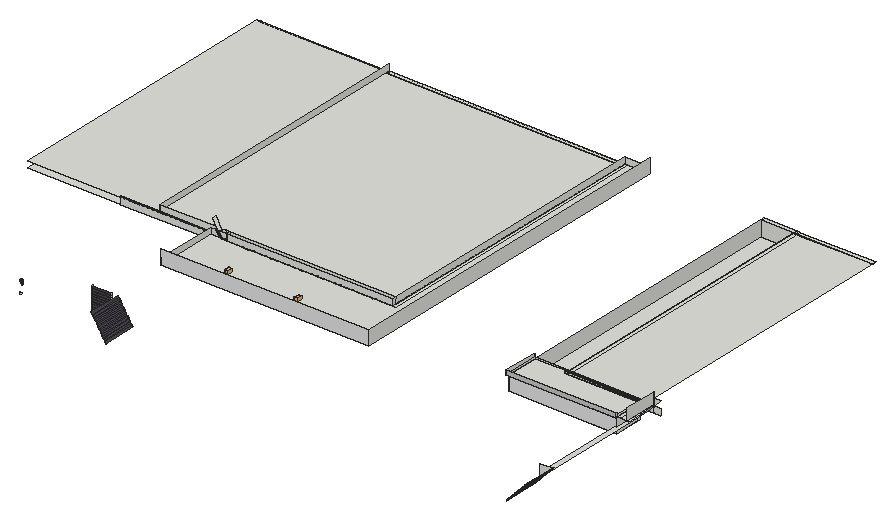
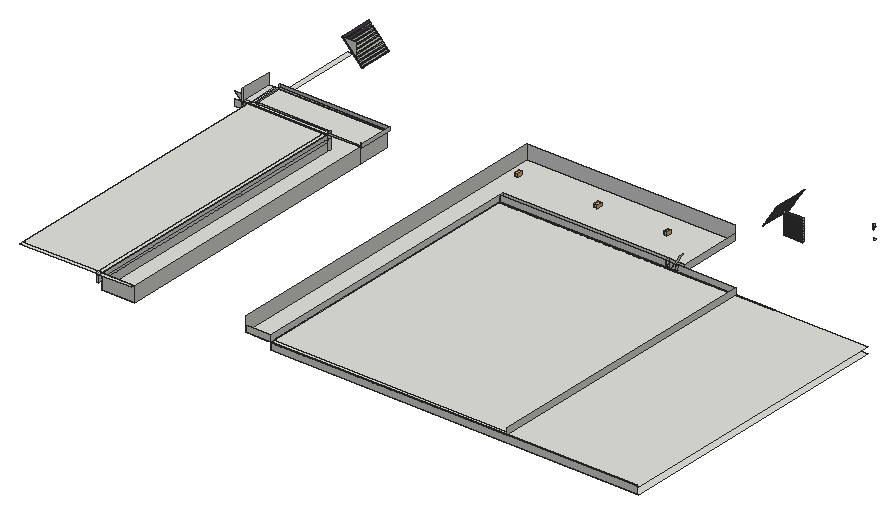
# SketchUp Ruby script. Lengths in inches.
U = 1.inch
M = Sketchup.active_model
def pt(a) = Geom::Point3d.new(a.map { |v| v * U })
def face(e, loops, mat)
  f = e.add_face(loops[0].map { |a| pt(a) })
  loops[1..].each { |l| e.add_face(l.map { |a| pt(a) }).erase! }
  f.material = f.back_material = mat if mat
  f
end
# faces: each face lists its corners as indices into pts; further lists are holes
def faces(e, pts, list, mat = nil) = list.each { |f| face(e, (f[0].is_a?(Array) ? f : [f]).map { |l| l.map { |i| pts[i] } }, mat) }
# xy, xz, yz: faces in a plane at the given z, y or x. An outline is a flat list of corners, or four numbers for a rectangle; further outlines are holes
def ring(l) = l.size == 4 ? [[l[0], l[1]], [l[2], l[1]], [l[2], l[3]], [l[0], l[3]]] : l.each_slice(2).to_a
def flat(e, list, mat, &to3) = list.each { |f| face(e, (f[0].is_a?(Array) ? f : [f]).map { |l| ring(l).map { |u, v| to3.(u, v) } }, mat) }
def xy(e, z, list, mat = nil) = flat(e, list, mat) { |x, y| [x, y, z] }
def xz(e, y, list, mat = nil) = flat(e, list, mat) { |x, z| [x, y, z] }
def yz(e, x, list, mat = nil) = flat(e, list, mat) { |y, z| [x, y, z] }
def lines(e, pts, list) = list.each { |a, b| e.add_line(pt(pts[a]), pt(pts[b])) }
# prism: a flat outline (further loops are holes) pulled along v
def prism(e, loops, v, mat = nil)
  f = face(e, loops, mat); d = Geom::Vector3d.new(v.map { |x| x * U })
  f.pushpull(f.normal.samedirection?(d) ? d.length : -d.length)
end
def box(e, o, s, mat = nil) = prism(e, [[o, [o[0] + s[0], o[1], o[2]], [o[0] + s[0], o[1] + s[1], o[2]], [o[0], o[1] + s[1], o[2]]]], [0, 0, s[2]], mat)
def at(x, y, z, deg = 0) = Geom::Transformation.translation(pt([x, y, z])) * Geom::Transformation.rotation(ORIGIN, Z_AXIS, deg.degrees)
def axes(o, x, y, z) = Geom::Transformation.new([*x, 0, *y, 0, *z, 0, *pt(o).to_a, 1])
def part(name) = M.definitions.add(name)
# library, detail: a bought-in or finely detailed component or shape, given as its bounding box
def library(name, o, s) = part(name).tap { |d| box(d.entities, o, s) }
def detail(e, o, s) = box(e.add_group.entities, o, s)
def put(e, d, t, mat = nil) = e.add_instance(d, t).tap { |i| i.material = mat if mat }
def group(e, t, mat = nil) = e.add_group.tap { |g| g.transformation = t; g.material = mat if mat }.entities
root = M.entities
M.materials.add("[Color M01]").color = [226, 226, 226]
M.materials.add("[Color M02]").color = [198, 198, 198]
M.materials.add("[Color M06]").color = [79, 71, 84]
c1 = library("Group\#13",[0,0,0],[3.54,3.54,3.9375])
xy(root,306.39,[[578.05,523.75,609.02,526.125]])
xy(root,307.2,[[578.05,523.75,609.02,526.125]])
xy(root,310.33,[[578.05,523.75,609.02,526.125]])
xy(root,311.14,[[578.05,523.75,609.02,526.125]])
xy(root,314.27,[[578.05,523.75,609.02,526.125]])
xy(root,315.08,[[578.05,524.25,609.02,526.125]])
xy(root,315.25,[[1139.11,678.64,1139.11,1195.68,1192.67,1195.68,1192.67,726.125,1316.04,726.125,1316.04,678.64]])
xy(root,318.2,[[578.05,524.25,609.02,526.125]])
xy(root,319.01,[[578.05,524.25,609.02,526.125]])
xy(root,322.14,[[578.05,524.25,609.02,526.125]])
xy(root,322.89,[[578.05,524.25,609.02,526.125]])
xy(root,326.02,[[578.05,524.25,609.02,526.125]])
xy(root,326.08,[[1314.46,528.48,1322.96,719.2],[1314.46,719.2,1322.96,719.59]])
xy(root,326.76,[[578.05,524.25,609.02,526.125]])
xy(root,328,[[306.21,732.2,910.57,1201.875]])
xy(root,329.89,[[578.05,524.25,609.02,526.125]])
xy(root,330.64,[[578.05,524.25,609.02,526.125]])
xy(root,333.125,[[1192.67,726.125,1196.48,732.2],[1192.67,732.2,1196.48,734.4375],[1192.67,734.4375,1196.48,1195.68]])
xy(root,333.71,[[497.26,480.14,499.58,480.77]])
xy(root,333.77,[[578.05,524.25,609.02,526.125]])
xy(root,334.51,[[578.05,524.25,609.02,526.125]])
xy(root,336.02,[[497.26,480.14,499.58,480.77]])
xy(root,336.52,[[497.26,480.14,499.58,480.77]])
xy(root,337.64,[[578.05,524.25,609.02,526.125]])
xy(root,338.39,[[578.05,524.25,609.02,526.125]])
xy(root,338.84,[[494.35,480.14,496.66,480.77],[497.26,480.14,499.58,480.77]])
xy(root,338.875,[[306.21,732.2,910.57,1201.875]])
xy(root,339.34,[[494.35,480.14,496.66,480.77],[497.26,480.14,499.58,480.77]])
xy(root,340.125,[[611.36,623.84,611.36,726.125,663.69,726.125,663.69,724.8125,669.77,724.8125,669.77,726.125,673.19,726.125,673.19,724.8125,679.27,724.8125,679.27,726.125,682.69,726.125,682.69,724.8125,688.77,724.8125,688.77,726.125,692.19,726.125,692.19,724.8125,698.27,724.8125,698.27,726.125,701.69,726.125,701.69,724.8125,707.77,724.8125,707.77,726.125,711.19,726.125,711.19,724.8125,717.27,724.8125,717.27,726.125,720.69,726.125,720.69,724.8125,726.77,724.8125,726.77,726.125,730.19,726.125,730.19,724.8125,736.27,724.8125,736.27,726.125,739.69,726.125,739.69,724.8125,745.77,724.8125,745.77,726.125,749.19,726.125,749.19,724.8125,755.27,724.8125,755.27,726.125,758.69,726.125,758.69,724.8125,764.77,724.8125,764.77,726.125,768.19,726.125,768.19,724.8125,774.27,724.8125,774.27,726.125,777.69,726.125,777.69,724.8125,783.77,724.8125,783.77,726.125,787.19,726.125,787.19,724.8125,793.27,724.8125,793.27,726.125,796.69,726.125,796.69,724.8125,802.77,724.8125,802.77,726.125,806.19,726.125,806.19,724.8125,812.27,724.8125,812.27,726.125,815.69,726.125,815.69,724.8125,821.77,724.8125,821.77,726.125,825.19,726.125,825.19,724.8125,831.27,724.8125,831.27,726.125,834.69,726.125,834.69,724.8125,840.77,724.8125,840.77,726.125,844.19,726.125,844.19,724.8125,850.27,724.8125,850.27,726.125,853.69,726.125,853.69,724.8125,859.77,724.8125,859.77,726.125,863.19,726.125,863.19,724.8125,869.27,724.8125,869.27,726.125,872.69,726.125,872.69,724.8125,878.77,724.8125,878.77,726.125,882.19,726.125,882.19,724.8125,888.27,724.8125,888.27,726.125,891.69,726.125,891.69,724.8125,897.77,724.8125,897.77,726.125,901.19,726.125,901.19,724.8125,907.27,724.8125,907.27,726.125,910.69,726.125,910.69,724.8125,916.77,724.8125,916.77,1201.875,952.01,1201.875,952.01,623.84],[1136.54,676.08,1139.11,678.64],[1139.11,676.08,1316.04,678.64],[1136.54,678.64,1139.11,732.2],[1139.11,678.64,1139.11,732.2,1192.67,732.2,1192.67,726.125,1316.04,726.125,1316.04,678.64],
  [1316.04,678.64,1322.24,726.125],[1322.24,678.64,1322.96,726.125],[1322.96,678.64,1333.34,726.125],[1333.34,678.64,1336.18,726.125],[663.69,724.8125,669.77,726.125],
  [673.19,724.8125,679.27,726.125],[682.69,724.8125,688.77,726.125],[692.19,724.8125,698.27,726.125],[701.69,724.8125,707.77,726.125],[711.19,724.8125,717.27,726.125],
  [720.69,724.8125,726.77,726.125],[730.19,724.8125,736.27,726.125],[739.69,724.8125,745.77,726.125],[749.19,724.8125,755.27,726.125],[758.69,724.8125,764.77,726.125],
  [768.19,724.8125,774.27,726.125],[777.69,724.8125,783.77,726.125],[787.19,724.8125,793.27,726.125],[796.69,724.8125,802.77,726.125],[806.19,724.8125,812.27,726.125],
  [815.69,724.8125,821.77,726.125],[825.19,724.8125,831.27,726.125],[834.69,724.8125,840.77,726.125],[844.19,724.8125,850.27,726.125],[853.69,724.8125,859.77,726.125],
  [863.19,724.8125,869.27,726.125],[872.69,724.8125,878.77,726.125],[882.19,724.8125,888.27,726.125],[891.69,724.8125,897.77,726.125],[901.19,724.8125,907.27,726.125],
  [910.69,724.8125,916.77,1201.875],[637.42,726.125,910.57,732.2],[910.57,726.125,910.69,732.2],[1192.67,726.125,1198.75,732.2],[1198.75,726.125,1322.24,732.2],
  [1322.96,726.125,1333.34,732.2],[1333.34,726.125,1336.18,732.2],[522.625,732.2,637.42,734.4375],[637.42,732.2,910.57,734.4375],[910.57,732.2,910.69,734.4375],
  [1192.67,732.2,1198.75,734.4375],[1198.75,732.2,1322.24,732.2,1322.24,732.32,1198.87,732.32,1198.87,734.4375,1198.75,734.4375],[1322.24,732.2,1322.96,734.4375],[1198.87,732.32,1322.24,734.4375],[522.625,734.4375,910.57,1195.68],
  [910.57,734.4375,910.69,1195.8],[1192.67,734.4375,1198.75,1195.68],[1198.75,734.4375,1198.87,1195.68],[1198.87,734.4375,1322.24,1195.68],[1322.24,734.4375,1322.96,1195.68],
  [522.625,1195.68,910.57,1195.8],[1139.11,1195.68,1192.67,1195.8],[1192.67,1195.68,1196.48,1195.8],[1192.67,1195.68,1196.48,1195.8],[1196.48,1195.68,1198.75,1195.8],
  [1198.75,1195.68,1322.24,1195.8],[1322.24,1195.68,1322.96,1195.8],[522.625,1195.8,910.57,1201.875],[910.57,1195.8,910.69,1201.875],[1139.11,1195.8,1192.67,1201.875],
  [1192.67,1195.8,1196.48,1201.875],[1196.48,1195.8,1198.75,1201.875],[1198.75,1195.8,1322.24,1201.875],[1322.24,1195.8,1322.96,1201.875]])
xz(root,480.7,[[494.35,319.65,496.66,321.96]])
xz(root,521.5625,[[646.07,305.32,646.4375,305.56,644.74,308.2,644.375,307.97],[1305.53,306.65,1305.08,307.08,1307.5,309.65,1307.95,309.22],[1305.08,307.08,1304.85,307.29,1307.27,309.87,1307.5,309.65],[643.84,308.8,644.21,309.03,642.52,311.68,642.15,311.44],[1308.83,310.16,1308.375,310.59,1310.8,313.16,1311.25,312.73],
  [641.62,312.27,641.98,312.51,640.29,315.15,639.92,314.91],[1312.13,313.66,1311.68,314.09,1314.1,316.66,1314.55,316.23],[639.39,315.74,639.76,315.98,638.0625,318.62,637.7,318.38],[1315.43,317.17,1314.97,317.59,1316.04,318.73,1316.04,317.82],[1316.04,317.82,1316.5,318.3,1316.04,318.73],
  [1316.5,318.3,1317.85,319.74,1317.39,320.17,1316.04,318.73],[1316.04,318.73,1317.39,320.17,1318.27,321.1,1320.69,323.67,1321.57,324.6,1322.96,326.08,1323.99,327.17,1324.87,328.11,1327.29,330.68,1328.17,331.61,1330.59,334.18,1331.47,335.11,1333.89,337.6875,1334.76,338.62,1336.18,340.125,1316.04,340.125],[637.16,319.21,637.53,319.45,635.84,322.09,635.47,321.86],[1318.73,320.67,1321.15,323.24,1320.69,323.67,1318.27,321.1],[634.9375,322.6875,635.31,322.92,633.61,325.57,633.24,325.33],
  [1322.03,324.17,1321.57,324.6,1322.96,326.08,1322.96,325.17],[1322.96,325.17,1322.96,326.08,1323.42,325.65],[1323.42,325.65,1324.45,326.75,1323.99,327.17,1322.96,326.08],[632.71,326.16,633.08,326.4,631.39,329.04,631.02,328.8],[1325.32,327.68,1327.75,330.25,1327.29,330.68,1324.87,328.11],
  [630.48,329.63,630.85,329.87,629.16,332.51,628.79,332.28],[1328.62,331.18,1331.04,333.75,1330.59,334.18,1328.17,331.61],[628.26,333.11,628.625,333.34,626.93,335.98,626.5625,335.75],[1331.92,334.6875,1334.34,337.26,1333.89,337.6875,1331.47,335.11],[626.03,336.58,626.4,336.8125,624.71,339.46,624.34,339.22],
  [1335.22,338.19,1336.64,339.7,1336.18,340.125,1334.76,338.62],[1336.64,339.7,1337.04,340.125,1336.18,340.125],[623.81,340.05,624.17,340.29,622.48,342.93,622.11,342.69],[1336.18,340.125,1337.04,340.125,1337.64,340.76,1337.1875,341.19]])
xz(root,523.75,[[578.05,307.2,609.02,310.33],[578.05,311.14,609.02,314.27]],"[Color M06]")
xz(root,524.25,[[578.05,315.08,609.02,318.2],[578.05,319.01,609.02,322.14],[578.05,322.89,609.02,326.02],[578.05,326.76,609.02,329.89],[578.05,330.64,609.02,333.77],
  [578.05,334.51,609.02,337.64],[578.05,338.39,609.02,341.52]],"[Color M06]")
xz(root,526.125,[[578.05,306.39,609.02,307.2],[578.05,310.33,609.02,311.14],[578.05,314.27,609.02,315.08],[578.05,318.2,609.02,319.01],[578.05,322.14,609.02,322.89],
  [578.05,326.02,609.02,326.76],[578.05,329.89,609.02,330.64],[578.05,333.77,609.02,334.51],[578.05,337.64,609.02,338.39]])
xz(root,623.84,[[611.36,340.125,952.01,363.75]],"[Color M01]")
xz(root,676.08,[[1136.54,340.125,1316.04,346.3125]],"[Color M02]")
xz(root,678.64,[[1139.11,340.125,1316.04,342.6875]])
xz(root,678.64,[[1139.11,315.25,1316.04,340.125]],"[Color M01]")
xz(root,726.125,[[1192.67,315.25,1196.48,333.125],[1196.48,315.25,1198.75,315.25,1198.75,340.125,1192.67,340.125,1192.67,333.125,1196.48,333.125],[1198.75,315.25,1310.86,340.125],[1310.86,315.25,1316.04,340.125],[611.36,340.125,611.36,350.1875,617.83,350.1875,624.28,340.125],
  [624.28,340.125,629.99,340.125,623.54,350.1875,617.83,350.1875],[629.99,340.125,623.54,350.1875,637.42,350.1875,637.42,340.125,635.26,343.5],[629.99,340.125,635.26,343.5,637.42,340.125],[637.42,340.125,910.57,350.1875],[1192.67,340.125,1198.75,342.6875],
  [1198.75,340.125,1310.86,342.6875],[1310.86,340.125,1316.04,342.6875]])
xz(root,732.2,[[1322.96,326.08,1322.96,328,1324.77,328],[459.19,328,617.83,338.875],[617.83,328,623.54,338.875],[623.54,328,630.97,328,630.97,329.69,625.08,338.875,623.54,338.875],[630.97,328,632.05,328,630.97,329.69],
  [632.05,328,637.42,328,637.42,338.875,630.97,338.875,630.97,329.69],[637.42,328,910.57,338.875],[1192.67,328,1198.75,338.875],[1198.75,328,1322.96,338.875],[1322.96,328,1322.96,338.875,1333.34,338.875,1333.34,337.11,1324.77,328],
  [1324.77,328,1333.34,328,1333.34,337.11],[1333.34,328,1345.65,328,1345.65,338.875,1335.01,338.875,1333.34,337.11],[630.97,329.69,630.97,338.875,625.08,338.875],[1333.34,337.11,1333.34,338.875,1335.01,338.875],[459.19,338.875,617.83,340.125],
  [617.83,338.875,623.54,340.125],[623.54,338.875,625.08,338.875,624.28,340.125,623.54,340.125],[625.08,338.875,630.97,338.875,630.97,340.125,624.28,340.125],[630.97,338.875,637.42,340.125],[637.42,338.875,910.57,340.125],
  [1192.67,338.875,1198.75,340.125],[1198.75,338.875,1322.96,340.125],[1322.96,338.875,1333.34,340.125],[1333.34,338.875,1333.34,340.125,1336.18,340.125,1335.01,338.875],[522.625,340.125,617.83,350.1875],
  [617.83,340.125,623.54,340.125,623.54,341.27,617.83,350.1875],[623.54,340.125,624.28,340.125,623.54,341.27],[624.28,340.125,629.99,340.125,623.54,350.1875,623.54,341.27],[629.99,340.125,630.97,340.75,630.97,350.1875,623.54,350.1875],[629.99,340.125,630.97,340.125,630.97,340.75],
  [630.97,340.125,637.42,340.125,637.42,350.1875,630.97,350.1875,635.26,343.5,630.97,340.75],[637.42,340.125,910.57,350.1875],[1136.54,340.125,1139.11,346.3125],[1139.11,340.125,1192.67,342.6875],[1333.34,340.125,1333.34,350.1875,1345.65,350.1875,1336.18,340.125]])
xz(root,1195.68,[[1139.11,315.25,1192.67,340.125],[1192.67,333.125,1196.48,340.125]])
xz(root,1201.875,[[310.02,328,910.57,338.875],[1192.67,328,1196.48,338.875],[310.02,338.875,910.57,340.125],[1192.67,338.875,1196.48,340.125],[910.57,340.125,952.01,350.1875]])
yz(root,496.66,[[480.14,336.52,480.77,338.84],[480.14,339.34,480.77,341.65]])
yz(root,497.26,[[480.14,336.52,480.77,338.84],[480.14,339.34,480.77,341.65]])
yz(root,499.58,[[480.14,336.52,480.77,338.84],[480.14,339.34,480.77,341.65]])
yz(root,522.625,[[732.2,340.125,1201.875,350.1875]])
yz(root,578.05,[[523.75,307.2,526.125,310.33],[523.75,311.14,526.125,314.27],[524.25,315.08,526.125,318.2],[524.25,319.01,526.125,322.14],[524.25,322.89,526.125,326.02],
  [524.25,326.76,526.125,329.89],[524.25,330.64,526.125,333.77],[524.25,334.51,526.125,337.64],[524.25,338.39,526.125,341.52]])
yz(root,609.02,[[523.75,307.2,526.125,310.33],[523.75,311.14,526.125,314.27],[524.25,315.08,526.125,318.2],[524.25,319.01,526.125,322.14],[524.25,322.89,526.125,326.02],
  [524.25,326.76,526.125,329.89],[524.25,330.64,526.125,333.77],[524.25,334.51,526.125,337.64],[524.25,338.39,526.125,341.52]])
yz(root,611.36,[[623.84,340.125,726.125,350.1875]])
yz(root,637.42,[[726.125,340.125,732.2,350.1875]])
yz(root,910.57,[[732.2,328,1195.68,338.875],[1195.68,328,1201.875,338.875],[732.2,338.875,1195.68,340.125],[1195.68,338.875,1201.875,340.125],[726.125,340.125,732.2,350.1875],
  [732.2,340.125,1201.875,350.1875]])
yz(root,952.01,[[623.84,340.125,1201.875,363.75]])
yz(root,1136.54,[[676.08,340.125,732.2,346.3125]])
yz(root,1139.11,[[678.64,315.25,732.2,340.125],[732.2,315.25,1195.68,340.125],[678.64,340.125,732.2,342.6875]])
yz(root,1192.67,[[726.125,315.25,732.2,333.125],[732.2,315.25,734.4375,328],[734.4375,315.25,1195.68,328],[732.2,328,734.4375,333.125],[734.4375,328,1195.68,333.125],
  [1195.68,328,1201.875,338.875],[726.125,333.125,732.2,340.125],[732.2,333.125,734.4375,338.875],[734.4375,333.125,1195.68,338.875],[732.2,338.875,734.4375,340.125],
  [734.4375,338.875,1195.68,340.125],[1195.68,338.875,1201.875,340.125],[726.125,340.125,732.2,342.6875]])
yz(root,1316.04,[[678.64,315.25,719.59,340.125],[719.59,315.25,726.125,340.125],[676.08,340.125,678.64,346.3125],[678.64,340.125,719.59,342.6875],[719.59,340.125,726.125,342.6875]])
yz(root,1322.96,[[726.125,326.08,732.2,340.125]])
yz(root,1333.34,[[678.64,340.125,731.75,358.5],[731.75,340.125,732.2,358.5]])
p = [[644.375,521.5625,307.97],[646.07,521.5625,305.32],[646.07,467.1875,305.32],[644.375,467.1875,307.97],[646.4375,521.5625,305.56],[646.4375,467.1875,305.56],
  [1304.2,521.5625,306.15],[1304.2,467.1875,306.15],[1304.66,467.1875,305.72],[1304.66,521.5625,305.72],[1303.97,521.5625,306.36],[1303.97,467.1875,306.36],
  [1305.08,521.5625,307.08],[1305.08,467.1875,307.08],[1305.53,521.5625,306.65],[1305.53,467.1875,306.65],[1307.95,521.5625,309.22],[1307.95,467.1875,309.22],
  [1304.85,467.1875,307.29],[1304.85,521.5625,307.29],[1307.5,521.5625,309.65],[1307.5,467.1875,309.65],[1307.27,521.5625,309.87],[1307.27,467.1875,309.87],
  [644.74,467.1875,308.2],[644.74,521.5625,308.2],[644.21,467.1875,309.03],[644.21,521.5625,309.03],[642.15,521.5625,311.44],[643.84,521.5625,308.8],
  [643.84,467.1875,308.8],[642.15,467.1875,311.44],[1308.375,521.5625,310.59],[1308.375,467.1875,310.59],[1308.83,521.5625,310.16],[1308.83,467.1875,310.16],
  [1311.25,521.5625,312.73],[1311.25,467.1875,312.73],[1310.8,521.5625,313.16],[1310.8,467.1875,313.16],[642.52,467.1875,311.68],[642.52,521.5625,311.68],
  [641.98,467.1875,312.51],[641.98,521.5625,312.51],[639.92,521.5625,314.91],[641.62,521.5625,312.27],[641.62,467.1875,312.27],[639.92,467.1875,314.91],
  [1311.68,521.5625,314.09],[1311.68,467.1875,314.09],[1312.13,521.5625,313.66],[1312.13,467.1875,313.66],[1314.55,521.5625,316.23],[1314.55,467.1875,316.23],
  [1314.1,521.5625,316.66],[1314.1,467.1875,316.66],[640.29,467.1875,315.15],[640.29,521.5625,315.15],[639.76,467.1875,315.98],[639.76,521.5625,315.98],
  [637.7,521.5625,318.38],[639.39,521.5625,315.74],[639.39,467.1875,315.74],[637.7,467.1875,318.38],[1314.97,521.5625,317.59],[1314.97,467.1875,317.59],
  [1315.43,521.5625,317.17],[1315.43,467.1875,317.17],[1316.5,521.5625,318.3],[1317.85,521.5625,319.74],[1317.85,467.1875,319.74],[1316.04,521.5625,317.82],
  [1317.39,521.5625,320.17],[1316.04,521.5625,318.73],[1317.39,467.1875,320.17],[638.0625,467.1875,318.62],[638.0625,521.5625,318.62],[637.53,467.1875,319.45],
  [637.53,521.5625,319.45],[635.47,521.5625,321.86],[637.16,521.5625,319.21],[637.16,467.1875,319.21],[635.47,467.1875,321.86],[1318.27,521.5625,321.1],
  [1318.27,467.1875,321.1],[1318.73,521.5625,320.67],[1318.73,467.1875,320.67],[1321.15,521.5625,323.24],[1321.15,467.1875,323.24],[1320.69,521.5625,323.67],
  [1320.69,467.1875,323.67],[635.84,467.1875,322.09],[635.84,521.5625,322.09],[635.31,467.1875,322.92],[635.31,521.5625,322.92],[633.24,521.5625,325.33],
  [634.9375,521.5625,322.6875],[634.9375,467.1875,322.6875],[633.24,467.1875,325.33],[1321.57,521.5625,324.6],[1321.57,467.1875,324.6],[1322.03,521.5625,324.17],
  [1322.03,467.1875,324.17],[1323.42,521.5625,325.65],[1324.45,521.5625,326.75],[1324.45,467.1875,326.75],[1322.96,521.5625,325.17],[1323.99,521.5625,327.17],
  [1322.96,521.5625,326.08],[1323.99,467.1875,327.17],[633.61,467.1875,325.57],[633.61,521.5625,325.57],[633.08,467.1875,326.4],[633.08,521.5625,326.4],
  [1322.96,719.59,326.08],[1322.96,719.2,326.08],[1312.29,719.2,336.13],[1312.29,731.75,336.13],[1322.96,731.75,326.08],[1322.96,726.125,326.08],
  [1336.18,719.59,340.125],[1336.18,726.125,340.125],[1336.18,731.75,340.125],[1336.18,732.2,340.125],[1335.01,732.2,338.875],[1333.34,732.2,337.11],
  [1324.77,732.2,328],[1322.96,732.2,326.08],[631.02,521.5625,328.8],[632.71,521.5625,326.16],[632.71,467.1875,326.16],[631.02,467.1875,328.8],
  [1324.87,521.5625,328.11],[1324.87,467.1875,328.11],[1325.32,521.5625,327.68],[1325.32,467.1875,327.68],[1327.75,521.5625,330.25],[1327.75,467.1875,330.25],
  [1327.29,521.5625,330.68],[1327.29,467.1875,330.68],[631.39,467.1875,329.04],[631.39,521.5625,329.04],[630.85,467.1875,329.87],[630.85,521.5625,329.87],
  [628.79,521.5625,332.28],[630.48,521.5625,329.63],[630.48,467.1875,329.63],[628.79,467.1875,332.28],[1328.17,521.5625,331.61],[1328.17,467.1875,331.61],
  [1328.62,521.5625,331.18],[1328.62,467.1875,331.18],[1331.04,521.5625,333.75],[1331.04,467.1875,333.75],[1330.59,521.5625,334.18],[1330.59,467.1875,334.18],
  [629.16,467.1875,332.51],[629.16,521.5625,332.51],[628.625,467.1875,333.34],[628.625,521.5625,333.34],[626.5625,521.5625,335.75],[628.26,521.5625,333.11],
  [628.26,467.1875,333.11],[626.5625,467.1875,335.75],[1331.47,521.5625,335.11],[1331.47,467.1875,335.11],[1331.92,521.5625,334.6875],[1331.92,467.1875,334.6875],
  [1334.34,521.5625,337.26],[1334.34,467.1875,337.26],[626.93,467.1875,335.98],[626.93,521.5625,335.98],[626.4,467.1875,336.8125],[626.4,521.5625,336.8125],
  [624.34,521.5625,339.22],[626.03,521.5625,336.58],[626.03,467.1875,336.58],[624.34,467.1875,339.22],[1333.89,521.5625,337.6875],[1333.89,467.1875,337.6875],
  [1334.76,521.5625,338.62],[1334.76,467.1875,338.62],[1335.22,521.5625,338.19],[1335.22,467.1875,338.19],[1337.04,521.5625,340.125],[1337.64,521.5625,340.76],
  [1337.64,467.1875,340.76],[1336.64,521.5625,339.7],[624.71,467.1875,339.46],[624.71,521.5625,339.46],[624.17,467.1875,340.29],[624.17,521.5625,340.29],
  [624.28,521.5625,340.125],[622.11,521.5625,342.69],[623.81,521.5625,340.05],[623.81,467.1875,340.05],[622.11,467.1875,342.69],[614.85,726.125,363.75],
  [614.09,726.125,364.9375],[614.09,732.2,364.9375],[623.54,732.2,350.1875],[629.99,732.2,340.125],[629.99,726.125,340.125],[623.54,726.125,350.1875],
  [617.83,726.125,359.1],[635.26,726.125,343.5],[630.97,732.2,340.75],[635.26,732.2,343.5],[1316.04,726.125,340.125],[1316.04,731.75,340.125],
  [1322.96,528.48,326.08],[1312.29,528.48,336.13],[629.99,521.5625,340.125]]
faces(root,p,[[0,1,2,3],[6,12,13,7],[13,12,14,15],[14,16,17,15],[24,26,27,25],[28,29,30,31],[20,32,33,21],[33,32,34,35],
  [34,36,37,35],[40,42,43,41],[44,45,46,47],[38,48,49,39],[50,52,53,51],[56,58,59,57],[60,61,62,63],[54,64,65,55],
  [68,69,70,67,66,71],[75,77,78,76],[79,80,81,82],[72,83,84,74],[85,87,88,86],[91,93,94,92],[95,96,97,98],[89,99,100,90],
  [103,104,105,102,101,106],[110,112,113,111],[128,129,130,131],[107,132,133,109],[134,136,137,135],[140,142,143,141],[144,145,146,147],[138,148,149,139],
  [150,152,153,151],[156,158,159,157],[160,161,162,163],[154,164,165,155],[166,168,169,167],[170,172,173,171],[174,175,176,177],[178,180,181,179],
  [184,185,186,183,182,187],[188,190,191,192,189],[193,194,195,196]],"[Color M06]")
faces(root,p,[[4,5,2,1],[6,7,8,9],[7,6,10,11],[12,13,18,19],[20,12,13,21],[22,19,18,23],[24,25,0,3],[27,26,30,29],
  [20,21,17,16],[21,20,22,23],[38,32,33,39],[40,41,28,31],[43,42,46,45],[38,39,37,36],[49,48,50,51],[54,48,49,55],
  [56,57,44,47],[59,58,62,61],[54,55,53,52],[65,64,66,67],[72,73,64,65,74],[75,76,60,63],[78,77,81,80],[72,74,70,69],
  [84,83,85,86],[89,83,84,90],[91,92,79,82],[94,93,97,96],[89,90,88,87],[100,99,101,102],[107,108,99,100,109],[110,111,95,98],
  [114,115,116,117,118,119],[114,120,121,122,118,119],[118,122,123,124,125,126,127],[113,112,130,129],[107,109,105,104],[133,132,134,135],[138,132,133,139],[140,141,128,131],
  [143,142,146,145],[138,139,137,136],[149,148,150,151],[154,148,149,155],[156,157,144,147],[159,158,162,161],[154,155,153,152],[165,164,166,167],
  [170,171,160,163],[173,172,176,175],[178,179,169,168],[181,180,182,183],[188,189,174,177],[191,190,195,194],[197,198,199,200,201,202,203,204],[205,202,201,206,207]])
lines(root,p,[[208,209],[210,211],[192,212]])
put(root,c1,axes([693.4,658.52,344.6875],[-1.5535,0,0],[0,2.39,0],[0,0,-3.63878]))
put(root,c1,axes([807.96,658.52,344.6875],[-1.5535,0,0],[0,2.39,0],[0,0,-3.63878]))
put(root,c1,axes([938.52,658.52,344.6875],[-1.5535,0,0],[0,2.39,0],[0,0,-3.63878]))
